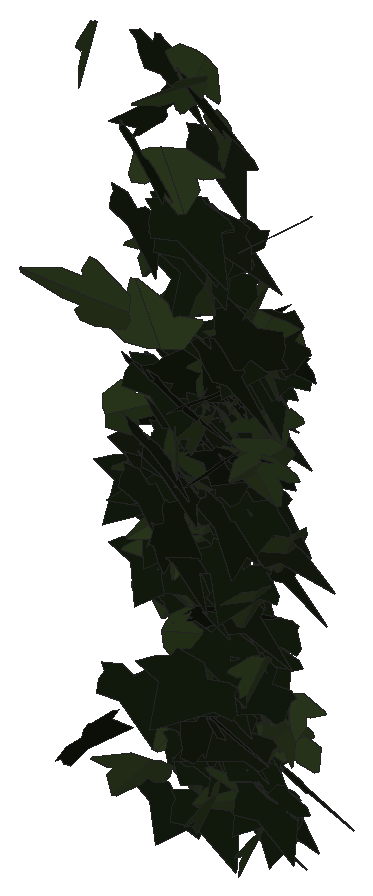
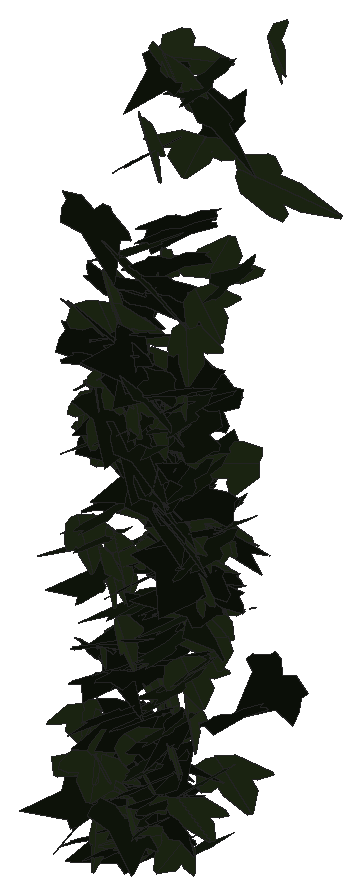
# SketchUp Ruby script. Lengths in millimetres.
U = 1.mm
M = Sketchup.active_model
def pt(a) = Geom::Point3d.new(a.map { |v| v * U })
def face(e, loops, mat)
  f = e.add_face(loops[0].map { |a| pt(a) })
  loops[1..].each { |l| e.add_face(l.map { |a| pt(a) }).erase! }
  f.material = f.back_material = mat if mat
  f
end
# faces: each face lists its corners as indices into pts; further lists are holes
def faces(e, pts, list, mat = nil) = list.each { |f| face(e, (f[0].is_a?(Array) ? f : [f]).map { |l| l.map { |i| pts[i] } }, mat) }
# xy, xz, yz: faces in a plane at the given z, y or x. An outline is a flat list of corners, or four numbers for a rectangle; further outlines are holes
def ring(l) = l.size == 4 ? [[l[0], l[1]], [l[2], l[1]], [l[2], l[3]], [l[0], l[3]]] : l.each_slice(2).to_a
def flat(e, list, mat, &to3) = list.each { |f| face(e, (f[0].is_a?(Array) ? f : [f]).map { |l| ring(l).map { |u, v| to3.(u, v) } }, mat) }
def xy(e, z, list, mat = nil) = flat(e, list, mat) { |x, y| [x, y, z] }
def xz(e, y, list, mat = nil) = flat(e, list, mat) { |x, z| [x, y, z] }
def yz(e, x, list, mat = nil) = flat(e, list, mat) { |y, z| [x, y, z] }
def lines(e, pts, list) = list.each { |a, b| e.add_line(pt(pts[a]), pt(pts[b])) }
# prism: a flat outline (further loops are holes) pulled along v
def prism(e, loops, v, mat = nil)
  f = face(e, loops, mat); d = Geom::Vector3d.new(v.map { |x| x * U })
  f.pushpull(f.normal.samedirection?(d) ? d.length : -d.length)
end
def box(e, o, s, mat = nil) = prism(e, [[o, [o[0] + s[0], o[1], o[2]], [o[0] + s[0], o[1] + s[1], o[2]], [o[0], o[1] + s[1], o[2]]]], [0, 0, s[2]], mat)
def at(x, y, z, deg = 0) = Geom::Transformation.translation(pt([x, y, z])) * Geom::Transformation.rotation(ORIGIN, Z_AXIS, deg.degrees)
def axes(o, x, y, z) = Geom::Transformation.new([*x, 0, *y, 0, *z, 0, *pt(o).to_a, 1])
def part(name) = M.definitions.add(name)
# library, detail: a bought-in or finely detailed component or shape, given as its bounding box
def library(name, o, s) = part(name).tap { |d| box(d.entities, o, s) }
def detail(e, o, s) = box(e.add_group.entities, o, s)
def put(e, d, t, mat = nil) = e.add_instance(d, t).tap { |i| i.material = mat if mat }
def group(e, t, mat = nil) = e.add_group.tap { |g| g.transformation = t; g.material = mat if mat }.entities
root = M.entities
M.materials.add("efeu1").color = [18, 25, 13]
M.materials.add("efeu2").color = [43, 57, 29]
c1 = part("ivyleaf_9")
p = [[39.1,54.8,31.7],[34.5,51.8,30.2],[-5.3,25.2,17.3],[-17.9,28.3,20.9],[-21.6,21.7,17],[-20.2,4.3,5.3],
  [-22.9,-0.3,2.5],[-17.1,-4,-0.6],[-2,-2.1,-1.2],[-0.7,-15.4,-10.1],[16.6,-22.3,-16.7],[21.1,-15.1,-12.5],
  [32.7,-10.7,-11],[46.1,-1.8,-6.6],[30.8,11.2,3.8]]
faces(c1.entities,p,[[0,1,2,3,4,5,6,7,8,9,10,11,12,13,14]],"efeu1")
c2 = part("ivyleaf_10")
p = [[0,12.8,-0.8],[-1.5,51.3,-10.9],[-4.9,51,-11.6],[-13.6,26.5,-7.3],[-13.2,15.9,-4.6],[-21.1,19.3,-7.2],
  [-29.5,16.3,-8.3],[-29.2,8.3,-6.2],[-19.7,-9.8,0.5],[-7.6,-13,4],[1,-12.2,5.8],[-0.4,51.1,-11.1],
  [-1.5,51.1,-10.9],[1,-12.4,5.9],[16.9,-12.4,3.5],[35.1,9.1,-5.1],[35,12.9,-6.1],[20.5,16.4,-4.9],
  [15.8,15,-3.8],[15.3,27.6,-7.1],[12.8,31.3,-7.8]]
faces(c2.entities,p,[[0,1,2,3,4,5,6,7,8,9,10],[11,12,0,13,14,15,16,17,18,19,20]],"efeu2")
put(root,c1,axes([1660.8,938.5,1756.5],[0.4415,-0.81167,-0.19024],[-0.02192,0.19433,-0.84315],[1.58647,0.22856,0.04129]))
put(root,c2,axes([1679.2,937.5,1994.9],[1.06332,-0.67737,-0.23325],[0.04542,0.31322,-0.85247],[1.3627,0.51811,0.21042]))
put(root,c1,axes([1655.6,930.7,2040.4],[0.97127,-0.76669,-0.01494],[0.08323,0.04701,-0.91889],[1.45707,0.50839,0.06244]))
put(root,c2,axes([1686.8,908.1,2043.1],[-0.971,-0.75326,0.02026],[-0.02427,-0.01584,-0.90978],[1.43392,-0.51035,-0.00167]))
put(root,c2,axes([1685.2,949.4,1721.5],[1.42051,0.331,-0.305],[-0.57981,-0.06325,-0.81416],[-0.63057,0.80381,0.06153]))
put(root,c2,axes([1688.1,942.1,1884.9],[-0.81079,-0.73898,0.20711],[-0.08482,-0.21265,-0.85045],[1.45815,-0.42327,0.06569]))
put(root,c1,axes([1675.8,916.5,2044.6],[-0.60653,-0.73457,0.46803],[-0.07183,-0.48626,-0.78888],[1.65614,-0.29011,0.13719]))
put(root,c2,axes([1662.9,870.7,2115.1],[0.07331,0.1013,-1.03408],[1.16357,0.83449,0.10452],[1.59892,-0.61192,-0.02865]))
put(root,c1,axes([1694.5,896.3,2032],[-1.69963,-0.19626,-0.10725],[0.20385,0.01224,-0.91428],[0.37366,-0.89937,0.01096]))
put(root,c1,axes([1684.6,907,1923.2],[0.56798,0.29509,0.82603],[0.27,0.8448,-0.35305],[-1.64742,0.2402,0.22692]))
put(root,c2,axes([1677.6,804,2595.7],[0.52642,-0.87809,0.5509],[0.58562,-0.47492,-0.91148],[1.88392,0.39299,0.1294]))
put(root,c1,axes([1670.3,893.7,2343.2],[0.16901,-0.88752,0.40494],[0.02757,-0.40537,-0.89164],[1.85644,0.08682,-0.02362]))
put(root,c1,axes([1680.5,940.5,2013.1],[1.34011,0.5638,-0.04726],[-0.0799,-0.02319,-0.902],[-1.07382,0.70534,0.00813]))
put(root,c1,axes([1673.2,938.4,1993],[-0.72011,-0.47497,-0.67524],[0.75573,0.54651,-0.60693],[1.37751,-0.54812,-0.02002]))
put(root,c2,axes([1692.1,898.6,1984.3],[0.83075,-0.7904,-0.01328],[-0.02813,0.00701,-0.90287],[1.50424,0.43665,-0.00955]))
put(root,c1,axes([1692.3,929.6,1973.4],[-0.90422,-0.7387,0.22055],[-0.15068,-0.21095,-0.87708],[1.45946,-0.47945,0.04609]))
put(root,c1,axes([1712.8,932.7,2043.3],[-0.22231,0.60112,0.68361],[-0.4231,0.64951,-0.60912],[-1.68004,-0.24311,0.06294]))
put(root,c1,axes([1678,934.6,2001.8],[-0.48068,-0.77284,-0.39845],[0.41662,0.34504,-0.808],[1.60155,-0.32171,0.0906]))
put(root,c2,axes([1672.3,916.1,1918.5],[-1.00811,0.37295,-0.64477],[0.99609,-0.3766,-0.6478],[-1.00869,-0.74463,0.00469]))
put(root,c2,axes([1698.1,903.3,2317.5],[-0.44009,-0.9054,0.24803],[-0.01114,-0.25404,-0.93283],[1.78662,-0.22461,0.05528]))
put(root,c2,axes([1701,911.9,1986.3],[0.37593,0.30725,-0.87481],[-0.77082,-0.776,-0.364],[-1.58738,0.44959,-0.03042]))
put(root,c2,axes([1697.8,904.6,1942.6],[1.30647,0.48259,-0.38033],[-0.63856,-0.18332,-0.8382],[-0.97967,0.76306,0.03916]))
put(root,c1,axes([1682.8,873.4,1799.8],[-0.17963,-0.86531,-0.13613],[0.01729,0.13594,-0.87043],[1.66703,-0.09465,-0.00564]))
put(root,c1,axes([1692.8,906.8,1931.1],[-0.82985,-0.69154,0.35139],[-0.04422,-0.39127,-0.79887],[1.47564,-0.40062,0.17366]))
put(root,c2,axes([1708.7,854.3,1715.6],[-1.05246,-0.67674,0.33486],[-0.42029,-0.25195,-0.87388],[1.37418,-0.59536,-0.01081]))
put(root,c1,axes([1672.3,939.2,1987.3],[0.73236,-0.81893,0.04314],[0.09522,-0.02412,-0.90416],[1.55784,0.38646,0.03499]))
put(root,c2,axes([1701,921.2,1824.6],[0.19035,-0.78517,-0.42269],[-0.10728,0.41892,-0.79151],[1.69371,0.11478,-0.00263]))
put(root,c1,axes([1665.8,936.3,1977.5],[1.44148,-0.43331,0.22126],[0.36978,-0.10596,-0.87257],[0.84892,0.78191,0.00437]))
put(root,c2,axes([1701.9,931.4,2005.2],[-0.98521,-0.70405,0.23317],[0.02448,-0.29283,-0.85563],[1.41131,-0.4864,0.17762]))
put(root,c2,axes([1706.1,930.8,2066.4],[-0.85464,-0.78383,0.16258],[-0.14486,-0.14377,-0.90333],[1.51663,-0.45543,0.00534]))
put(root,c1,axes([1684,914.6,2096.1],[1.49694,0.45963,0.17256],[0.2679,0.10108,-0.91085],[-0.89516,0.79888,0.01597]))
put(root,c1,axes([1684.1,932.4,1881.7],[0.2445,-0.86186,0.21474],[0.04959,-0.21322,-0.87136],[1.68971,0.13097,-0.0055]))
put(root,c1,axes([1680.1,917.1,2115.1],[0.98118,-0.76888,-0.16119],[-0.10906,0.15548,-0.92492],[1.49117,0.51729,0.03842]))
put(root,c1,axes([1684.9,945.6,1881.6],[0.25898,-0.85215,0.19138],[0.04703,-0.18986,-0.86293],[1.66155,0.1382,-0.00541]))
put(root,c1,axes([1681.8,956.8,1874.5],[0.73613,-0.7726,-0.13519],[0.01693,0.15505,-0.86062],[1.49266,0.37927,0.07643]))
put(root,c1,axes([1705.7,759.9,1789.1],[-0.31379,0.31858,-1.017],[-0.78699,0.92935,0.35816],[1.86939,0.44472,-0.01993]))
put(root,c1,axes([1699.3,918.3,1642.4],[-0.48933,-0.68546,0.53173],[-0.12746,-0.53725,-0.72497],[1.64614,-0.24536,0.10192]))
put(root,c1,axes([1697.1,938.5,2041.6],[-0.48303,-0.87101,-0.03018],[-0.00136,0.03164,-0.90718],[1.65869,-0.25362,-0.00953]))
put(root,c1,axes([1719.4,912.1,2017.7],[0.39708,0.14702,0.91682],[-1.5908,-0.37949,0.25107],[0.7696,-0.86027,0.04593]))
put(root,c1,axes([1689,938.2,1969.3],[0.27068,-0.86709,-0.16141],[0.03701,0.16654,-0.8775],[1.67818,0.13618,0.04539]))
put(root,c1,axes([1707,930.6,1807.2],[0.34647,-0.07427,-0.86937],[-0.91363,0.73307,-0.16315],[1.38669,0.50155,0.10972]))
put(root,c2,axes([1702.6,941.3,1664.3],[-1.37597,0.49216,-0.18339],[0.27976,-0.10994,-0.87456],[-0.95965,-0.73772,0.00799]))
put(root,c1,axes([1690.4,937.9,1947.6],[0.62821,-0.79042,-0.25721],[-0.03986,0.26875,-0.85276],[1.58146,0.32075,0.08068]))
put(root,c1,axes([1692.2,960,1818.5],[0.4824,-0.82244,-0.09754],[-0.00279,0.10156,-0.86015],[1.57624,0.25188,0.02833]))
put(root,c2,axes([1683,932.9,2025.2],[-0.19837,-0.07776,-0.90568],[1.25031,-0.63651,-0.02095],[-1.19573,-0.65267,0.12834]))
put(root,c2,axes([1698.7,899.8,2040.5],[-1.46582,-0.17374,-0.47536],[0.92286,-0.00534,-0.7837],[0.27594,-0.90505,0.09587]))
put(root,c1,axes([1707.2,934.6,1887.5],[-0.61369,-0.82781,0.14276],[0.04168,-0.16115,-0.88497],[1.5982,-0.31366,0.0779]))
put(root,c1,axes([1702.4,954.6,1703.5],[-0.83767,0.03671,-0.72642],[1.3731,-0.08569,-0.44147],[-0.17563,-0.84502,0.01322]))
put(root,c1,axes([1693.9,932.3,2022.5],[1.27023,-0.61661,-0.10554],[-0.12499,0.08441,-0.90849],[1.18402,0.67042,0.01732]))
put(root,c2,axes([1721.1,899,2263.1],[-0.47066,-0.89571,-0.26018],[0.09673,0.25583,-0.92904],[1.77254,-0.2518,-0.01839]))
put(root,c1,axes([1702.6,872.8,2035],[0.08309,-0.8872,0.30401],[0.00337,-0.30426,-0.88818],[1.78489,0.04187,-0.01248]))
put(root,c2,axes([1721.6,927.6,1784.2],[0.22449,-0.87056,-0.15486],[-0.00534,0.15586,-0.87833],[1.68285,0.11663,0.01787]))
put(root,c1,axes([1687.9,911.4,2159.8],[1.43334,-0.52571,0.14139],[0.37022,0.03445,-0.90803],[0.96768,0.7655,0.13796]))
put(root,c1,axes([1731.6,932.1,2076.2],[0.11951,0.91278,-0.01474],[-0.10815,-0.01084,-0.91322],[-1.73405,0.06358,0.05594]))
put(root,c1,axes([1701.3,948.7,1852.2],[0.54028,-0.89558,-0.14098],[-0.04909,0.13969,-0.93933],[1.72475,0.28452,0.01742]))
put(root,c1,axes([1705,905.5,2058],[0.16608,-0.9231,0.08257],[0.03408,-0.08124,-0.92716],[1.76353,0.0885,0.01014]))
put(root,c1,axes([1703.3,946.6,1908.7],[0.71327,-0.79034,-0.14379],[-0.06367,0.14317,-0.87415],[1.52753,0.37501,0.03071]))
put(root,c1,axes([1751.3,901.3,2039.3],[-1.61191,-0.15141,0.42886],[-0.77912,-0.1411,-0.85829],[0.37708,-0.93879,0.05984]))
put(root,c1,axes([1696.7,924.4,2108.3],[0.90704,-0.755,0.24779],[0.29123,-0.19633,-0.89252],[1.48402,0.49999,0.0237]))
put(root,c1,axes([1735.7,945.5,1729.5],[0.89358,0.00828,0.71979],[-1.3659,-0.06104,0.46885],[0.10589,-0.85722,-0.02643]))
put(root,c1,axes([1710.1,918.7,2077.2],[0.09383,-0.91653,-0.07833],[0.04919,0.07979,-0.91736],[1.75,0.0469,0.02998]))
put(root,c2,axes([1723.9,900.5,1977.6],[0.34289,0.82699,-0.40912],[-0.22074,-0.39324,-0.84596],[-1.74206,0.2126,0.02667]))
put(root,c1,axes([1745.8,926.3,2092.7],[-0.51674,0.88535,-0.03982],[-0.02703,-0.04598,-0.92565],[-1.68648,-0.27053,0.02703]))
put(root,c1,axes([1705.6,911.4,2180.2],[1.00873,-0.76026,-0.21882],[-0.10047,0.22881,-0.92285],[1.50231,0.52578,0.08521]))
put(root,c1,axes([1714.5,940.4,1712.2],[-0.05794,-0.7035,-0.54291],[0.04883,0.54231,-0.70415],[1.69053,-0.03978,0.00173]))
put(root,c1,axes([1751.4,836.3,2517.9],[-0.88529,0.90858,0.01759],[-0.01517,0.01568,-1.02073],[-1.72946,-0.46522,-0.00005]))
put(root,c2,axes([1724.3,930.7,2062.8],[1.17371,0.68403,0.02259],[-0.12084,0.08746,-0.91491],[-1.29694,0.61089,0.10569]))
put(root,c2,axes([1738.3,895.6,2170.9],[-1.0618,0.6618,0.41279],[-0.52944,0.30531,-0.86546],[-1.38683,-0.62325,0.01436]))
put(root,c2,axes([1764.5,895.9,2028.8],[0.16227,0.10533,-0.92906],[-1.72177,0.24501,-0.05524],[0.44963,0.90021,0.12374]))
put(root,c1,axes([1747.9,922.9,2073.8],[-1.52711,0.33823,-0.27243],[0.39895,-0.19964,-0.86525],[-0.7239,-0.82353,0.09786]))
put(root,c1,axes([1714.4,938.1,1690.9],[0.42378,-0.78651,-0.31242],[0.05514,0.32995,-0.80998],[1.6097,0.19575,0.11]))
put(root,c1,axes([1720.9,880.1,2174.8],[-0.27959,-0.96307,-0.15309],[0.04524,0.15124,-0.97421],[1.85538,-0.14881,0.00068]))
put(root,c1,axes([1708.9,866,2094.7],[0.34965,-0.73858,0.56581],[0.41391,-0.52666,-0.7581],[1.72167,0.27661,0.06735]))
put(root,c2,axes([1737.1,911.1,2008],[-1.16282,-0.66415,-0.12514],[0.2567,0.04547,-0.89989],[1.26038,-0.62201,0.06783]))
put(root,c2,axes([1780,708.1,2353.1],[0.02581,0.05992,1.19884],[-2.25525,-0.19054,0.02293],[0.36433,-1.18368,0.05699]))
put(root,c1,axes([1715.8,866.9,2567.1],[0.74205,-0.93612,0.00333],[-0.02845,-0.00984,-1.01392],[1.78141,0.38978,-0.01758]))
put(root,c1,axes([1702.9,868.5,2166.5],[1.04685,-0.5863,0.62123],[0.79906,-0.45791,-0.80391],[1.4158,0.69195,-0.00563]))
put(root,c1,axes([1723.1,960.5,1766.3],[0.51661,-0.81931,0.02453],[0.01207,-0.02374,-0.8631],[1.55996,0.27151,-0.00145]))
put(root,c1,axes([1715.7,950,1725.4],[0.84069,-0.65348,0.37756],[0.38539,-0.31881,-0.7887],[1.38369,0.48583,-0.00972]))
put(root,c1,axes([1758.1,961.9,1681.8],[0.23846,0.79836,0.29937],[-0.16326,0.31285,-0.79841],[-1.61451,0.08628,0.12495]))
put(root,c2,axes([1751,901.3,1829.6],[0.3209,-0.88368,-0.08123],[-0.03134,0.07955,-0.89962],[1.68862,0.16941,-0.00126]))
put(root,c1,axes([1731.3,904.7,1935.1],[0.19696,-0.84045,-0.29216],[0.0496,0.29686,-0.84476],[1.69272,0.08909,0.05875]))
put(root,c1,axes([1743.8,917.9,2193.2],[-0.80148,-0.82982,0.15585],[0.06693,-0.19125,-0.92327],[1.60553,-0.40627,0.11629]))
put(root,c2,axes([1751.5,955.6,1692.7],[0.22682,-0.84197,-0.10734],[0.01062,0.10917,-0.85011],[1.61537,0.1175,0.02066]))
put(root,c1,axes([1737.9,953.6,1728.5],[-0.16363,-0.85654,0.06344],[-0.00776,-0.06335,-0.86085],[1.63462,-0.08604,0.00226]))
put(root,c1,axes([1736,928.2,1647.2],[-0.15978,-0.8203,-0.28988],[0.13362,0.28389,-0.82368],[1.6504,-0.1024,0.03862]))
put(root,c2,axes([1762.7,909.7,2060.6],[-1.10819,-0.63775,0.3283],[-0.37119,-0.26616,-0.86295],[1.31372,-0.61318,0.03312]))
put(root,c2,axes([1751.2,926.1,2097],[-0.90606,0.77088,0.19871],[-0.20627,0.16662,-0.90603],[-1.501,-0.48823,0.00456]))
put(root,c2,axes([1756.3,947.6,1774.2],[-0.60131,-0.54289,0.58824],[-0.04553,-0.62572,-0.59033],[1.52278,-0.23308,0.21463]))
put(root,c2,axes([1754.8,911,2006.9],[-0.49131,-0.83034,0.27287],[0.04813,-0.2915,-0.86311],[1.66276,-0.23691,0.10561]))
put(root,c1,axes([1783.9,927.3,1754.5],[-1.4114,0.06419,0.53106],[-1.00606,0.05109,-0.74435],[-0.15592,-0.9107,-0.00433]))
put(root,c2,axes([1734.7,874.5,2112.9],[0.67248,-0.64675,0.74932],[0.96011,-0.56689,-0.72717],[1.62084,0.60413,0.11985]))
put(root,c2,axes([1733.6,948.8,1663.1],[0.21579,-0.19335,-0.83228],[1.03016,0.66588,-0.08095],[1.25826,-0.51201,0.20901]))
put(root,c1,axes([1730,916.8,2144.4],[0.77934,-0.84435,-0.11484],[0.01136,0.13025,-0.93637],[1.62171,0.40485,0.06175]))
put(root,c1,axes([1733.4,923.2,1999.7],[0.23774,-0.82781,-0.32581],[0.18808,0.33988,-0.82567],[1.68264,0.07897,0.13833]))
put(root,c1,axes([1731.5,871.3,2067.3],[0.14135,-0.79347,0.61327],[0.32442,-0.59601,-0.79178],[1.88083,0.16243,0.09049]))
put(root,c2,axes([1750.5,900.3,2143.2],[0.90604,-0.79399,0.25862],[0.21599,-0.23342,-0.92551],[1.57452,0.48891,-0.02186]))
put(root,c1,axes([1758,918.3,2117.3],[0.73684,0.78249,0.28941],[-0.0055,0.32032,-0.86217],[-1.58783,0.36201,0.13729]))
put(root,c1,axes([1730.5,927,2095.5],[1.68038,-0.25971,0.02898],[0.08634,0.05178,-0.9182],[0.48979,0.88188,0.06244]))
put(root,c1,axes([1734.2,939.4,1749.2],[0.97251,-0.59355,-0.38575],[-0.01489,0.47099,-0.73507],[1.34717,0.43368,0.27035]))
put(root,c1,axes([1749.8,955.6,1864.7],[-0.58401,-0.80497,-0.14554],[0.04367,0.14692,-0.86094],[1.55625,-0.3062,-0.03046]))
put(root,c1,axes([1755.3,897,1730.2],[-0.44907,-0.3809,0.88967],[1.04496,0.7014,0.44591],[-1.51676,0.596,0.0438]))
put(root,c1,axes([1722.7,913.9,1773.1],[1.2016,-0.60151,0.43671],[0.59473,-0.30511,-0.87201],[1.28361,0.70445,-0.00478]))
put(root,c1,axes([1773.6,899.3,2292.1],[-1.69909,-0.32041,0.09017],[-0.11948,-0.09139,-0.94631],[0.62212,-0.89263,0.06452]))
put(root,c2,axes([1749.8,898,2071.5],[-1.4668,-0.34323,-0.36147],[0.70069,0.05674,-0.83886],[0.63954,-0.84937,0.09003]))
put(root,c2,axes([1736.7,870.3,1876.5],[0.35688,-0.56593,-0.73593],[0.80796,-0.61542,0.58143],[-1.57131,-0.44498,0.13182]))
put(root,c1,axes([1775.8,924.6,2131.4],[-0.4129,0.90548,-0.00616],[0.02565,-0.00311,-0.93102],[-1.72315,-0.21702,-0.01238]))
put(root,c1,axes([1740.7,951.9,1683.1],[0.94878,-0.68551,-0.13966],[-0.11616,0.12822,-0.84723],[1.32639,0.50158,0.0257]))
put(root,c1,axes([1760.4,827.5,2031.4],[0.52576,-0.36518,-0.96289],[-1.10018,0.77007,-0.4579],[1.62204,0.64068,0.00153]))
put(root,c1,axes([1748,881.4,2378.5],[-0.09151,-0.95101,-0.24874],[0.03986,0.24799,-0.95219],[1.87043,-0.05181,0.00812]))
put(root,c2,axes([1765.2,913.7,1837.7],[0.31992,-0.85845,0.10884],[0.01056,-0.10981,-0.87461],[1.64685,0.16747,-0.01554]))
put(root,c1,axes([1741,935.4,1753],[0.91218,-0.75573,-0.05224],[-0.04075,0.04828,-0.89487],[1.44117,0.4797,0.00777]))
put(root,c2,axes([1756.1,914.5,2150.4],[-1.263,0.59101,-0.30182],[0.30018,-0.27414,-0.8836],[-1.2268,-0.67552,0.09452]))
put(root,c1,axes([1744.6,907.7,2132.7],[0.41068,-0.9131,0.06439],[0.01442,-0.06437,-0.93822],[1.74207,0.21579,-0.00741]))
put(root,c1,axes([1786.4,917.9,2201.4],[-1.00357,0.77765,-0.02322],[0.02236,-0.02009,-0.93957],[-1.48052,-0.52744,0.00155]))
put(root,c1,axes([1785.9,904.5,2069.5],[-1.63808,0.30878,-0.06585],[0.09689,-0.05298,-0.91383],[-0.59301,-0.86159,0.0326]))
put(root,c1,axes([1751.6,893.7,2346],[-0.30118,-0.9116,-0.31859],[0.15364,0.30922,-0.92489],[1.83142,-0.17585,0.0252]))
put(root,c1,axes([1745.3,810.2,2470.1],[0.07827,-0.61141,0.89089],[0.21497,-0.88422,-0.61205],[2.04516,0.11634,0.03024]))
put(root,c1,axes([1750.1,934,1800.4],[0.20266,-0.83522,-0.26526],[0.02122,0.26848,-0.84088],[1.66769,0.09808,0.04293]))
put(root,c1,axes([1754.2,926.8,1934.7],[-0.21712,-0.81287,0.38841],[0.06757,-0.39526,-0.81679],[1.71326,-0.08743,0.08144]))
put(root,c2,axes([1753,943.9,1743.5],[0.89181,-0.4986,0.5259],[0.71188,-0.36999,-0.68406],[1.1813,0.59937,0.01521]))
put(root,c1,axes([1749.6,892.2,1888.8],[1.08103,0.40342,0.70098],[0.99462,0.47066,-0.69434],[-1.17475,0.76973,0.05718]))
put(root,c1,axes([1752.2,923.5,1969.3],[0.45267,-0.82499,-0.31362],[-0.0255,0.32139,-0.85561],[1.67956,0.22723,0.07153]))
put(root,c1,axes([1759.1,973.7,1654.4],[-0.09076,-0.83724,-0.05007],[-0.00551,0.05031,-0.83858],[1.59627,-0.04743,-0.00574]))
put(root,c2,axes([1773.5,791.1,2278.8],[1.45184,0.74931,0.11152],[-0.15984,-0.07364,1.06928],[1.43291,-0.76742,0.00628]))
put(root,c2,axes([1758.2,831.3,2459.7],[1.40348,0.69098,0.18934],[0.24627,0.13879,-1.01049],[-1.34113,0.74859,0.01258]))
put(root,c2,axes([1790.4,835.3,2557.3],[-0.31091,0.40857,-0.92125],[-1.19915,-0.76979,-0.22967],[-1.49693,0.5318,0.37532]))
put(root,c1,axes([1783.1,865.6,2173.3],[0.13434,0.94602,0.02335],[-0.00849,0.02374,-0.94863],[-1.801,0.07045,0.00622]))
put(root,c1,axes([1755.2,866.9,2384.6],[0.01621,-0.90825,-0.39058],[0.12657,0.39023,-0.906],[1.87738,-0.01847,0.06446]))
put(root,c1,axes([1751.4,929.7,1781.8],[1.23577,0.38049,0.49242],[0.77119,0.2816,-0.75191],[-0.89886,0.76471,0.03188]))
put(root,c1,axes([1784.3,897.9,2308.7],[-1.48304,-0.54246,0.1085],[-0.14655,-0.07924,-0.94923],[1.0426,-0.78275,0.0209]))
put(root,c2,axes([1777.2,941.5,1902],[0.14585,-0.8776,-0.04927],[-0.01243,0.04889,-0.88093],[1.67282,0.07688,-0.00225]))
put(root,c1,axes([1781,947.2,1714.9],[-1.17599,-0.57593,0.17462],[-0.18833,-0.14963,-0.84369],[1.1298,-0.62442,0.04112]))
put(root,c2,axes([1803.6,920.1,1682],[-0.97478,-0.28882,0.75947],[-1.28332,-0.34982,-0.58778],[0.86282,-0.84661,-0.01622]))
put(root,c1,axes([1796.7,919.7,1755.9],[-1.73339,-0.05074,0.10069],[-0.19094,-0.00921,-0.91218],[0.0979,-0.91628,0.00359]))
put(root,c2,axes([1779.7,868.5,2143.1],[-0.03098,-0.94355,-0.0167],[0.00081,0.01669,-0.9437],[1.79605,-0.01628,0.00014]))
put(root,c1,axes([1756.7,920.1,2017.7],[0.71887,-0.72988,-0.37118],[-0.1203,0.38156,-0.81461],[1.55377,0.36723,0.10866]))
put(root,c2,axes([1774.4,861.2,2564.8],[1.65263,-0.61453,-0.01149],[-0.01766,0.00678,-1.0638],[1.16965,0.86839,0.00017]))
put(root,c1,axes([1804.2,907.1,2333.5],[-1.0287,0.74449,0.27635],[-0.34959,0.20802,-0.91966],[-1.47039,-0.57031,0.02531]))
put(root,c1,axes([1772.9,896.1,2204.3],[0.74836,0.67448,0.53432],[0.38776,0.49778,-0.77829],[-1.59109,0.43855,0.06164]))
put(root,c1,axes([1758.1,848.3,1997.1],[0.41028,-0.86108,0.23473],[0.04493,-0.23589,-0.88703],[1.698,0.2143,-0.03324]))
put(root,c2,axes([1782.2,894.4,2204.5],[-0.24636,-0.90458,0.32863],[0.00838,-0.33215,-0.91251],[1.83167,-0.12015,0.04838]))
put(root,c1,axes([1746,865.6,2178.5],[0.28303,-0.0125,1.04738],[1.92955,0.26756,-0.14076],[-0.50096,1.02349,0.04959]))
put(root,c1,axes([1803.3,921.4,1848.5],[0.17967,0.21642,-0.88082],[-1.69404,0.19234,-0.04814],[0.33184,0.86473,0.23115]))
put(root,c1,axes([1768.4,895,1872.3],[-0.2159,-0.81154,-0.36458],[0.249,0.34832,-0.81605],[1.67482,-0.1564,0.07433]))
put(root,c2,axes([1785.7,918.3,2153.8],[0.833,-0.74713,-0.32841],[0.06644,0.38946,-0.83948],[1.55182,0.38437,0.21223]))
put(root,c1,axes([1768.5,958.5,1811.4],[0.40586,-0.71466,-0.43865],[0.04865,0.45794,-0.73367],[1.59518,0.16787,0.13398]))
put(root,c2,axes([1784.3,948.6,1763.5],[-0.56452,-0.7641,-0.46343],[0.42872,0.4086,-0.81787],[1.64588,-0.36851,0.05409]))
put(root,c1,axes([1797.7,844.2,1851.9],[-1.43207,-0.58306,0.12384],[-0.18942,-0.07374,-0.95191],[1.11851,-0.759,-0.00265]))
put(root,c1,axes([1780,943.4,1854.3],[-0.4642,-0.85401,0.12371],[-0.01311,-0.12663,-0.88772],[1.64226,-0.2424,0.02788]))
put(root,c1,axes([1765.5,943.1,1644.7],[1.48591,-0.38751,0.00067],[0.00147,0.00004,-0.87162],[0.73751,0.78074,0.00038]))
put(root,c2,axes([1792.5,968.4,1743.6],[-1.39035,-0.429,-0.07664],[0.11345,0.04982,-0.84709],[0.8216,-0.73285,-0.01272]))
put(root,c2,axes([1793.9,879.4,2485.3],[0.95692,-0.78984,-0.35606],[-0.17624,0.36033,-0.93007],[1.63947,0.49975,0.10784]))
put(root,c1,axes([1803.8,900.4,2100.6],[-0.8161,0.51904,-0.66568],[0.37974,-0.66316,-0.64561],[-1.56099,-0.43268,0.19096]))
put(root,c1,axes([1779.2,915.1,2219.6],[0.32937,0.23053,0.90145],[1.0249,0.72292,-0.28826],[-1.44413,0.56564,0.00102]))
put(root,c2,axes([1793.1,963.8,1658.1],[-0.04596,-0.69176,-0.48275],[0.0789,0.48139,-0.69188],[1.6035,-0.04352,0.02021]))
put(root,c2,axes([1792.8,920.3,2162.1],[-1.30764,0.63251,0.03574],[-0.13641,-0.02522,-0.93148],[-1.19798,-0.68754,0.06705]))
put(root,c1,axes([1766.1,894.9,2362.3],[0.78476,-0.81669,-0.35429],[0.15311,0.42304,-0.88153],[1.68736,0.34144,0.24476]))
put(root,c2,axes([1792.7,927.4,1996.1],[1.25052,-0.55162,-0.29941],[-0.11834,0.37413,-0.82573],[1.18865,0.61758,0.23279]))
put(root,c2,axes([1796.7,855.2,1705.3],[0.18136,-1.02806,-0.19432],[-0.04076,0.19317,-1.03247],[1.99084,0.09761,-0.00344]))
put(root,c1,axes([1794.9,921.2,2153.4],[0.6554,0.81979,0.29721],[0.04748,0.31016,-0.8844],[-1.65891,0.33276,0.09211]))
put(root,c1,axes([1768,898.4,2157.7],[1.69483,0.2495,0.27417],[0.48249,0.11062,-0.92408],[-0.51475,0.92517,0.03655]))
put(root,c2,axes([1792.7,851.4,2311.3],[0.1831,-0.84611,-0.48465],[0.26154,0.49391,-0.835],[1.83727,0.01401,0.16716]))
put(root,c1,axes([1771.4,913.1,2159.5],[1.27748,-0.64743,-0.0718],[-0.09876,0.04962,-0.93258],[1.2358,0.67323,-0.00031]))
put(root,c1,axes([1781.5,889,2464.9],[0.14588,-0.98925,-0.02502],[-0.03664,0.0236,-0.99206],[1.88299,0.0771,-0.01737]))
put(root,c1,axes([1801.2,951.7,1879.8],[-1.02101,-0.61708,0.31627],[-0.14958,-0.34318,-0.80291],[1.31118,-0.51966,0.15468]))
put(root,c2,axes([1801.1,911.7,2192.7],[-1.1387,-0.67527,-0.26229],[0.2815,0.21914,-0.90158],[1.34967,-0.61542,-0.03325]))
put(root,c1,axes([1781.6,936.5,1721],[0.37813,-0.79225,-0.3372],[0.09915,0.35649,-0.80687],[1.63569,0.16154,0.12686]))
put(root,c2,axes([1796.6,918.2,2178.8],[1.75248,-0.16105,-0.05798],[-0.02996,0.23625,-0.90616],[0.32438,0.89187,0.22957]))
put(root,c1,axes([1788.9,838.3,2550.5],[1.48892,-0.42719,-0.51522],[-0.78709,0.31458,-0.8888],[1.00149,0.88233,0.06745]))
put(root,c1,axes([1790.4,942.9,1840.4],[-0.21109,-0.78383,-0.37772],[0.13986,0.37097,-0.79141],[1.65004,-0.13172,0.01876]))
put(root,c2,axes([1808.5,932.3,1972.7],[0.8772,-0.62283,-0.4477],[-0.20997,0.46305,-0.75776],[1.44466,0.44549,0.16171]))
put(root,c1,axes([1815.3,886.1,2099.6],[0.90487,0.57943,-0.60516],[-0.70438,-0.47899,-0.7494],[-1.43054,0.60236,-0.01379]))
put(root,c1,axes([1809,944.5,1678.3],[-1.0223,-0.60991,0.24873],[-0.15217,-0.2582,-0.8058],[1.24432,-0.53266,0.10581]))
put(root,c2,axes([1819.9,964.1,1735.1],[1.09209,0.24443,-0.58515],[-1.07102,-0.16753,-0.62182],[-0.55639,0.80225,0.04844]))
put(root,c2,axes([1803.1,959,1746.9],[0.91441,-0.69593,0.14974],[0.18082,-0.11635,-0.84559],[1.34268,0.48962,0.0119]))
put(root,c1,axes([1785.9,926.4,2138.3],[0.82175,-0.70131,-0.42947],[-0.02243,0.47974,-0.79525],[1.56496,0.37513,0.21411]))
put(root,c2,axes([1810.5,902.1,2191.7],[0.41867,-0.91822,0.11871],[0.01913,-0.11964,-0.94404],[1.76201,0.21948,-0.01796]))
put(root,c2,axes([1817,891.6,2240.5],[-1.57241,-0.45765,0.09285],[-0.14583,-0.05327,-0.94443],[0.8767,-0.82969,0.00943]))
put(root,c1,axes([1807.3,897.7,1966.2],[-0.80911,-0.8034,0.19731],[-0.11344,-0.19151,-0.90823],[1.57037,-0.42778,0.03605]))
put(root,c1,axes([1788,903.2,1916.2],[0.80684,-0.76707,-0.2839],[-0.02181,0.31417,-0.86596],[1.55652,0.40202,0.13503]))
put(root,c2,axes([1815.6,926.6,2133.7],[-0.373,-0.89751,0.1172],[0.00336,-0.12029,-0.91825],[1.72263,-0.1941,0.02717]))
put(root,c1,axes([1804.9,960.9,1647],[-0.47919,-0.78578,0.22303],[-0.06095,-0.22371,-0.82432],[1.55337,-0.25118,0.03646]))
put(root,c1,axes([1811.7,905.4,2232.6],[-0.98061,-0.78089,0.17721],[-0.05231,-0.19336,-0.93195],[1.52308,-0.5094,0.08209]))
put(root,c1,axes([1824.8,915,2230.2],[1.08065,0.30967,-0.69401],[-1.16247,-0.32952,-0.64676],[-0.8606,0.83395,0.00215]))
put(root,c1,axes([1836.6,901.6,1835.7],[-1.88555,0.12903,-0.01038],[0.01851,-0.0057,-0.99908],[-0.24566,-0.99077,0.00439]))
put(root,c1,axes([1794.1,940.9,2037.1],[0.65843,-0.81009,-0.20481],[-0.00716,0.22016,-0.87716],[1.59026,0.3364,0.08085]))
put(root,c1,axes([1809,910.2,2035.7],[-0.6089,-0.86118,0.0712],[-0.03458,-0.0692,-0.91867],[1.64423,-0.32037,0.00704]))
put(root,c2,axes([1831.3,908.7,2258.3],[-1.59436,-0.33257,0.30291],[-0.35542,-0.32539,-0.87372],[0.77888,-0.82925,0.22136]))
put(root,c1,axes([1805.8,877.1,2027.5],[-0.06088,-0.80115,0.61232],[-0.04217,-0.61192,-0.80178],[1.91863,-0.03887,0.00181]))
put(root,c1,axes([1820.7,921.2,2211.8],[-1.14573,-0.70882,-0.12277],[0.2002,0.07163,-0.92936],[1.3544,-0.6102,0.03351]))
put(root,c2,axes([1825.5,903.3,2295.5],[0.39299,-0.94188,-0.09465],[0.03425,0.10076,-0.96346],[1.8013,0.20357,0.03897]))
put(root,c2,axes([1824.5,894.8,1649.3],[0.2588,-0.85125,0.13331],[0.07921,-0.12832,-0.8618],[1.63794,0.14071,0.02061]))
put(root,c2,axes([1829.2,885,1944.6],[-0.43517,-0.88154,-0.0035],[0.00225,0.00331,-0.91071],[1.67775,-0.22865,0.00032]))
put(root,c2,axes([1833.1,928.7,1766.9],[1.06252,-0.45123,-0.54294],[-0.45779,0.5292,-0.68714],[1.2632,0.57132,0.20766]))
put(root,c1,axes([1815.7,948.4,1667.5],[0.68931,-0.5327,-0.55435],[-0.60644,0.45366,-0.64413],[1.33161,0.48236,-0.00639]))
put(root,c2,axes([1824.8,899.7,1854],[-0.17341,-0.80566,0.38234],[0.24333,-0.39217,-0.79589],[1.6797,-0.02637,0.15477]))
put(root,c2,axes([1817.9,903.2,2225.7],[-1.08896,0.73013,-0.19511],[0.27948,-0.13265,-0.92702],[-1.41092,-0.58979,-0.03304]))
put(root,c2,axes([1827.2,922.7,2172.4],[0.40183,-0.85345,-0.31342],[0.05548,0.32795,-0.87338],[1.72946,0.18777,0.10084]))
put(root,c1,axes([1803.3,946.6,1955.5],[0.92684,-0.74696,0.00794],[0.08361,0.01918,-0.89043],[1.41923,0.48668,0.04728]))
put(root,c1,axes([1846.1,859,2247.3],[0.59661,0.13519,0.89793],[-1.02101,0.794,0.06774],[-1.39436,-0.52356,0.3346]))
put(root,c1,axes([1803.8,970.2,1692.8],[1.26589,-0.52089,0.04945],[0.16785,0.03278,-0.84103],[0.98156,0.66617,0.08005]))
put(root,c2,axes([1825.5,889.3,2102.4],[-1.68763,-0.05479,-0.25274],[0.48906,-0.08491,-0.88314],[0.05548,-0.91813,0.09676]))
put(root,c1,axes([1816.4,918.9,2195.3],[0.07253,-0.92513,0.18372],[0.0122,-0.18361,-0.92592],[1.79505,0.03863,-0.00113]))
put(root,c2,axes([1829.7,947.6,1787.1],[0.5081,0.83917,-0.04994],[-0.23028,-0.01349,-0.87359],[-1.58328,0.27127,0.11103]))
put(root,c2,axes([1846.3,897.5,2117],[-0.5456,-0.62588,0.62813],[-0.37852,-0.59793,-0.68657],[1.64461,-0.34526,0.05036]))
put(root,c1,axes([1809.9,928.1,1996.8],[0.86282,-0.68545,-0.36424],[0.11619,0.452,-0.77461],[1.47272,0.36592,0.27451]))
put(root,c2,axes([1833.7,907.4,2147.4],[-1.02292,-0.74461,-0.18774],[0.3296,0.10572,-0.91509],[1.42384,-0.55942,0.07696]))
put(root,c1,axes([1822.6,921.7,1688.9],[-0.13398,-0.82612,-0.27403],[0.00687,0.27465,-0.8289],[1.6565,-0.06795,-0.01873]))
put(root,c1,axes([1847.9,902.5,2374],[-0.03448,0.96729,0.05748],[0.00094,0.0575,-0.96746],[-1.8442,-0.01806,-0.00157]))
put(root,c1,axes([1861.3,910.4,2248.7],[-1.63127,0.41957,0.01544],[-0.01759,0.01625,-0.95424],[-0.79887,-0.8571,-0.01053]))
put(root,c1,axes([1813.3,842.5,2245.9],[0.97805,-0.90185,-0.06053],[-0.04868,0.0551,-1.03798],[1.71958,0.51451,0.00505]))
put(root,c2,axes([1843,928.3,1998.2],[-0.42778,-0.8951,-0.03345],[-0.00649,0.03534,-0.92281],[1.70474,-0.22448,-0.01191]))
